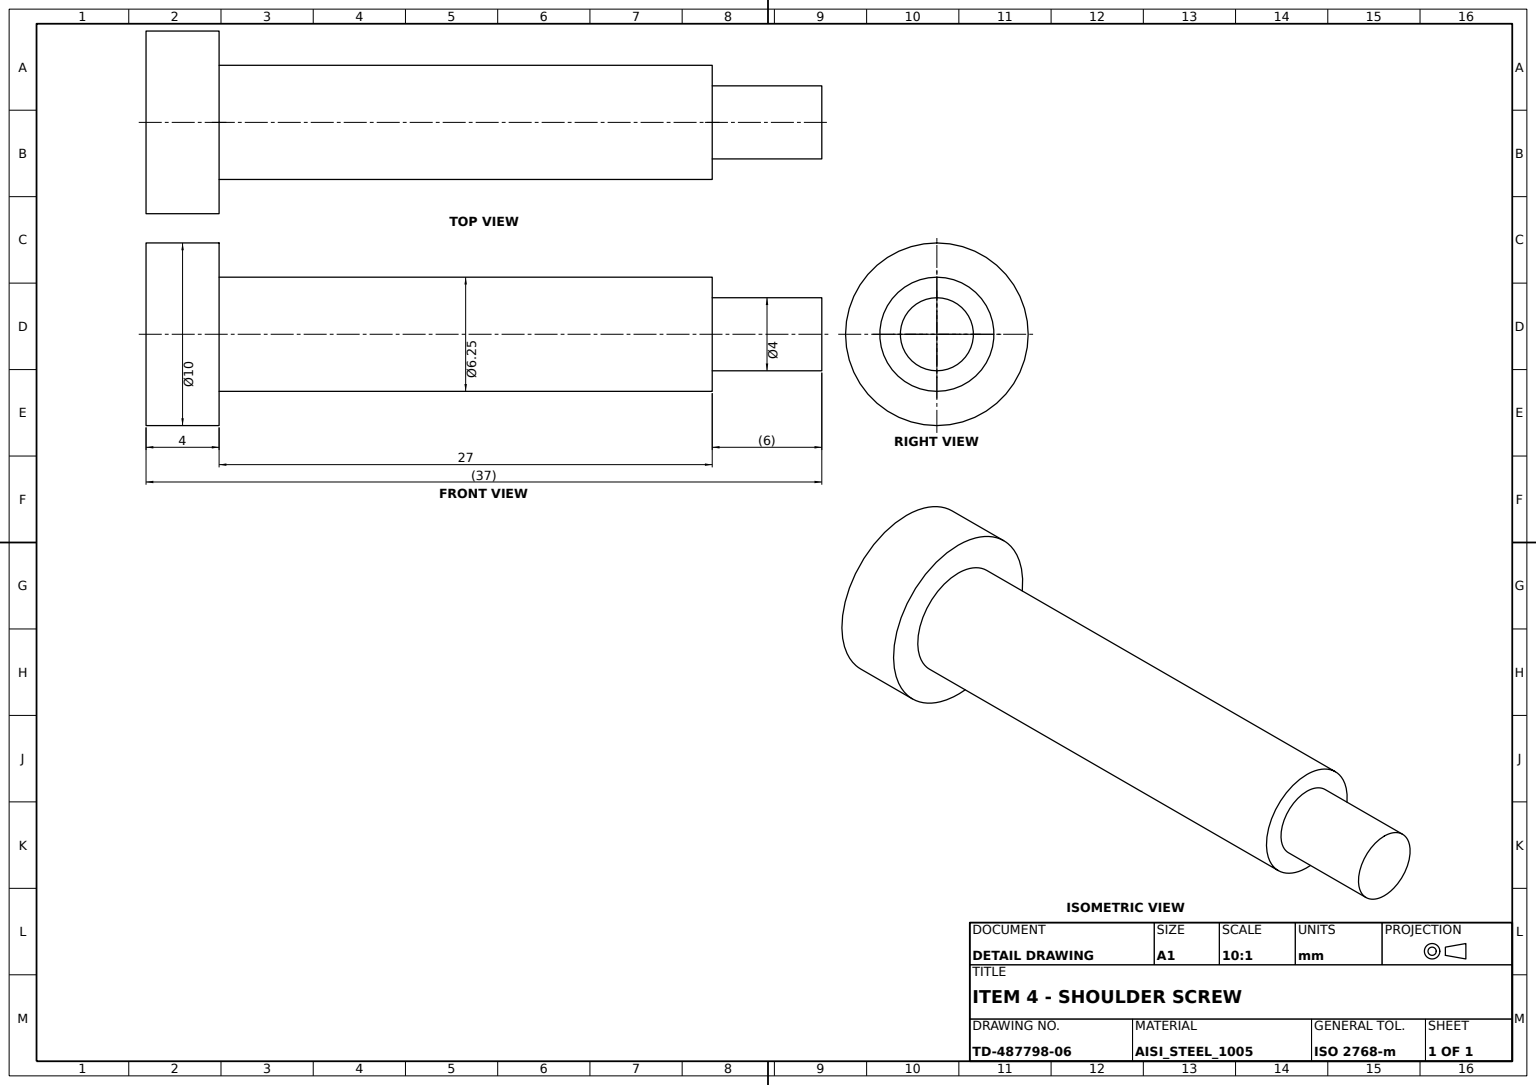
ISO-10303-21;
HEADER;
FILE_DESCRIPTION((''),'2;1');
FILE_NAME('','',(''),(''),'','','');
FILE_SCHEMA(('AUTOMOTIVE_DESIGN'));
ENDSEC;
DATA;
#1=APPLICATION_CONTEXT('');
#2=PRODUCT_CONTEXT('',#1,'mechanical');
#3=PRODUCT('','','',(#2));
#4=PRODUCT_DEFINITION_FORMATION('','',#3);
#5=PRODUCT_DEFINITION_CONTEXT('',#1,'design');
#6=PRODUCT_DEFINITION('','',#4,#5);
#7=PRODUCT_DEFINITION_SHAPE('','',#6);
#8=(LENGTH_UNIT()NAMED_UNIT(*)SI_UNIT(.MILLI.,.METRE.));
#9=(NAMED_UNIT(*)PLANE_ANGLE_UNIT()SI_UNIT($,.RADIAN.));
#10=(NAMED_UNIT(*)SI_UNIT($,.STERADIAN.)SOLID_ANGLE_UNIT());
#11=UNCERTAINTY_MEASURE_WITH_UNIT(LENGTH_MEASURE(0.005),#8,'distance_accuracy_value','');
#12=(GEOMETRIC_REPRESENTATION_CONTEXT(3)GLOBAL_UNCERTAINTY_ASSIGNED_CONTEXT((#11))GLOBAL_UNIT_ASSIGNED_CONTEXT((#8,#9,#10))REPRESENTATION_CONTEXT('',''));
#13=CARTESIAN_POINT('',(37.,0.,5.));
#14=VERTEX_POINT('',#13);
#15=CARTESIAN_POINT('',(37.,0.,0.));
#16=DIRECTION('',(-1.,0.,0.));
#17=DIRECTION('',(0.,0.,1.));
#18=AXIS2_PLACEMENT_3D('',#15,#16,#17);
#19=CIRCLE('',#18,5.);
#20=EDGE_CURVE('',#14,#14,#19,.T.);
#21=ORIENTED_EDGE('',*,*,#20,.F.);
#22=EDGE_LOOP('',(#21));
#23=FACE_BOUND('',#22,.T.);
#24=DIRECTION('',(1.,0.,0.));
#25=DIRECTION('',(0.,0.,-1.));
#26=AXIS2_PLACEMENT_3D('',#13,#24,#25);
#27=PLANE('',#26);
#28=ADVANCED_FACE('',(#23),#27,.T.);
#29=CARTESIAN_POINT('',(33.,0.,5.));
#30=VERTEX_POINT('',#29);
#31=CARTESIAN_POINT('',(33.,0.,0.));
#32=AXIS2_PLACEMENT_3D('',#31,#16,#17);
#33=CIRCLE('',#32,5.);
#34=EDGE_CURVE('',#30,#30,#33,.T.);
#35=ORIENTED_EDGE('',*,*,#34,.T.);
#36=EDGE_LOOP('',(#35));
#37=FACE_BOUND('',#36,.T.);
#38=CARTESIAN_POINT('',(33.,0.,3.125));
#39=VERTEX_POINT('',#38);
#40=CIRCLE('',#32,3.125);
#41=EDGE_CURVE('',#39,#39,#40,.T.);
#42=ORIENTED_EDGE('',*,*,#41,.F.);
#43=EDGE_LOOP('',(#42));
#44=FACE_BOUND('',#43,.T.);
#45=AXIS2_PLACEMENT_3D('',#38,#16,#17);
#46=PLANE('',#45);
#47=ADVANCED_FACE('',(#37,#44),#46,.T.);
#48=CARTESIAN_POINT('',(6.,0.,3.125));
#49=VERTEX_POINT('',#48);
#50=CARTESIAN_POINT('',(6.,0.,0.));
#51=AXIS2_PLACEMENT_3D('',#50,#16,#17);
#52=CIRCLE('',#51,3.125);
#53=EDGE_CURVE('',#49,#49,#52,.T.);
#54=ORIENTED_EDGE('',*,*,#53,.T.);
#55=EDGE_LOOP('',(#54));
#56=FACE_BOUND('',#55,.T.);
#57=CARTESIAN_POINT('',(6.,0.,2.));
#58=VERTEX_POINT('',#57);
#59=CIRCLE('',#51,2.);
#60=EDGE_CURVE('',#58,#58,#59,.T.);
#61=ORIENTED_EDGE('',*,*,#60,.F.);
#62=EDGE_LOOP('',(#61));
#63=FACE_BOUND('',#62,.T.);
#64=AXIS2_PLACEMENT_3D('',#57,#16,#17);
#65=PLANE('',#64);
#66=ADVANCED_FACE('',(#56,#63),#65,.T.);
#67=ORIENTED_EDGE('',*,*,#34,.F.);
#68=EDGE_LOOP('',(#67));
#69=FACE_BOUND('',#68,.T.);
#70=ORIENTED_EDGE('',*,*,#20,.T.);
#71=EDGE_LOOP('',(#70));
#72=FACE_BOUND('',#71,.T.);
#73=CARTESIAN_POINT('',(0.,0.,0.));
#74=AXIS2_PLACEMENT_3D('',#73,#16,#17);
#75=CYLINDRICAL_SURFACE('',#74,5.);
#76=ADVANCED_FACE('',(#69,#72),#75,.T.);
#77=CARTESIAN_POINT('',(0.,0.,2.));
#78=VERTEX_POINT('',#77);
#79=CIRCLE('',#74,2.);
#80=EDGE_CURVE('',#78,#78,#79,.T.);
#81=ORIENTED_EDGE('',*,*,#80,.T.);
#82=EDGE_LOOP('',(#81));
#83=FACE_BOUND('',#82,.T.);
#84=PLANE('',#74);
#85=ADVANCED_FACE('',(#83),#84,.T.);
#86=ORIENTED_EDGE('',*,*,#60,.T.);
#87=EDGE_LOOP('',(#86));
#88=FACE_BOUND('',#87,.T.);
#89=ORIENTED_EDGE('',*,*,#80,.F.);
#90=EDGE_LOOP('',(#89));
#91=FACE_BOUND('',#90,.T.);
#92=CYLINDRICAL_SURFACE('',#74,2.);
#93=ADVANCED_FACE('',(#88,#91),#92,.T.);
#94=ORIENTED_EDGE('',*,*,#53,.F.);
#95=EDGE_LOOP('',(#94));
#96=FACE_BOUND('',#95,.T.);
#97=ORIENTED_EDGE('',*,*,#41,.T.);
#98=EDGE_LOOP('',(#97));
#99=FACE_BOUND('',#98,.T.);
#100=CYLINDRICAL_SURFACE('',#74,3.125);
#101=ADVANCED_FACE('',(#96,#99),#100,.T.);
#102=CLOSED_SHELL('',(#28,#47,#66,#76,#85,#93,#101));
#103=MANIFOLD_SOLID_BREP('',#102);
#104=ADVANCED_BREP_SHAPE_REPRESENTATION('',(#103),#12);
#105=SHAPE_DEFINITION_REPRESENTATION(#7,#104);
ENDSEC;
END-ISO-10303-21;
